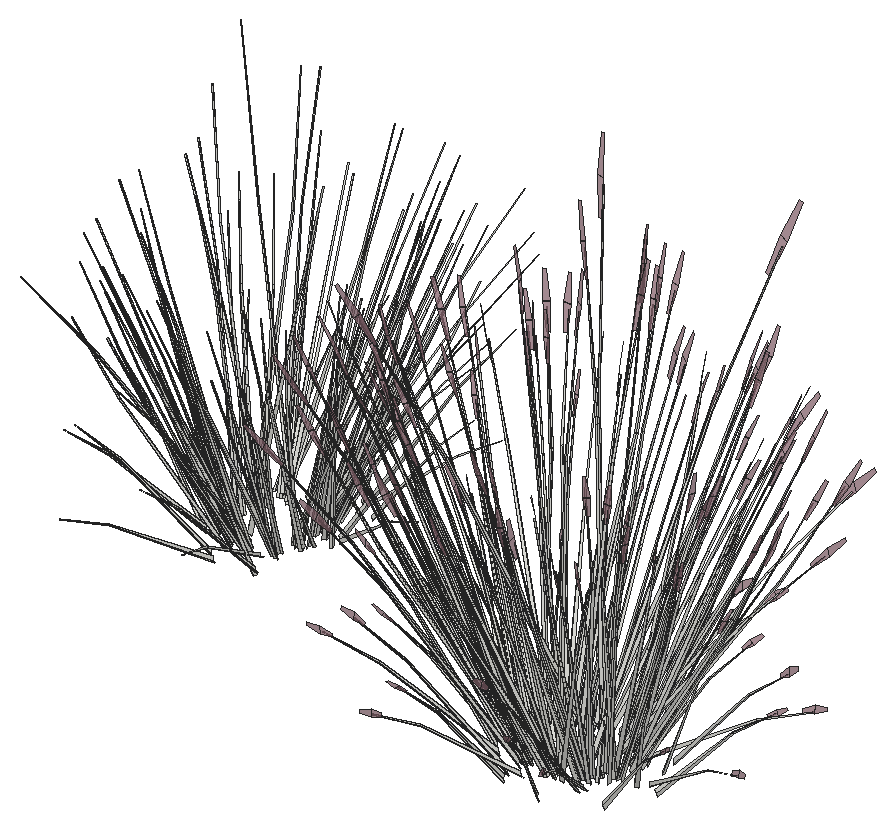
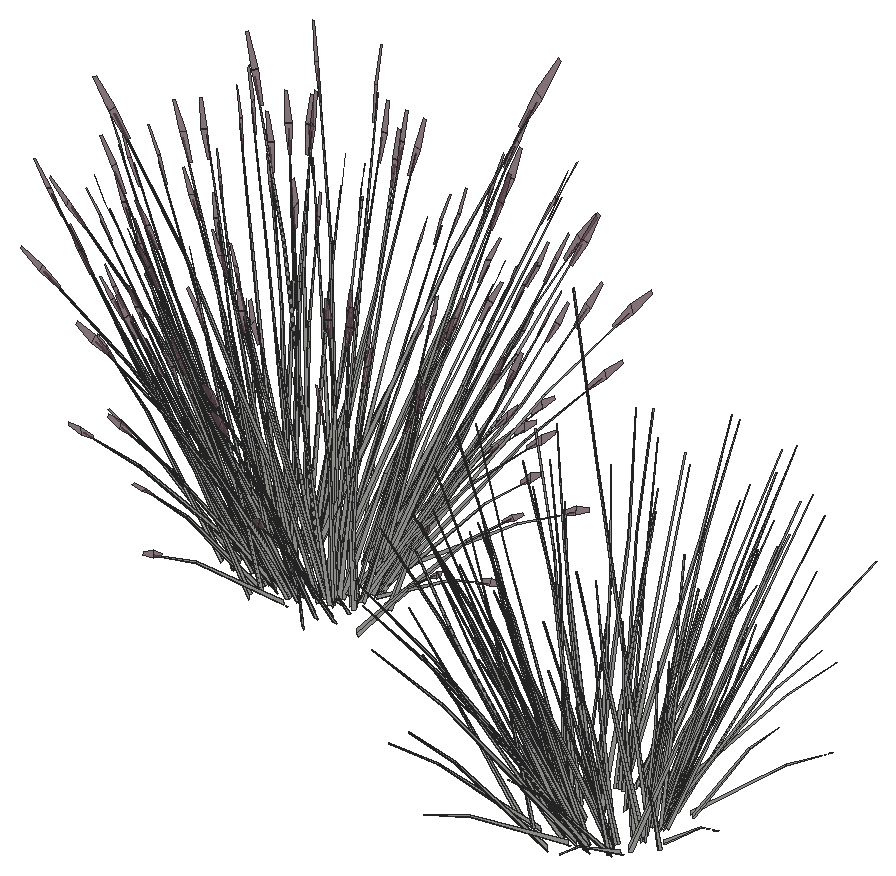
# SketchUp Ruby script. Lengths in inches.
U = 1.inch
M = Sketchup.active_model
def pt(a) = Geom::Point3d.new(a.map { |v| v * U })
def face(e, loops, mat)
  f = e.add_face(loops[0].map { |a| pt(a) })
  loops[1..].each { |l| e.add_face(l.map { |a| pt(a) }).erase! }
  f.material = f.back_material = mat if mat
  f
end
# faces: each face lists its corners as indices into pts; further lists are holes
def faces(e, pts, list, mat = nil) = list.each { |f| face(e, (f[0].is_a?(Array) ? f : [f]).map { |l| l.map { |i| pts[i] } }, mat) }
# xy, xz, yz: faces in a plane at the given z, y or x. An outline is a flat list of corners, or four numbers for a rectangle; further outlines are holes
def ring(l) = l.size == 4 ? [[l[0], l[1]], [l[2], l[1]], [l[2], l[3]], [l[0], l[3]]] : l.each_slice(2).to_a
def flat(e, list, mat, &to3) = list.each { |f| face(e, (f[0].is_a?(Array) ? f : [f]).map { |l| ring(l).map { |u, v| to3.(u, v) } }, mat) }
def xy(e, z, list, mat = nil) = flat(e, list, mat) { |x, y| [x, y, z] }
def xz(e, y, list, mat = nil) = flat(e, list, mat) { |x, z| [x, y, z] }
def yz(e, x, list, mat = nil) = flat(e, list, mat) { |y, z| [x, y, z] }
def lines(e, pts, list) = list.each { |a, b| e.add_line(pt(pts[a]), pt(pts[b])) }
# prism: a flat outline (further loops are holes) pulled along v
def prism(e, loops, v, mat = nil)
  f = face(e, loops, mat); d = Geom::Vector3d.new(v.map { |x| x * U })
  f.pushpull(f.normal.samedirection?(d) ? d.length : -d.length)
end
def box(e, o, s, mat = nil) = prism(e, [[o, [o[0] + s[0], o[1], o[2]], [o[0] + s[0], o[1] + s[1], o[2]], [o[0], o[1] + s[1], o[2]]]], [0, 0, s[2]], mat)
def at(x, y, z, deg = 0) = Geom::Transformation.translation(pt([x, y, z])) * Geom::Transformation.rotation(ORIGIN, Z_AXIS, deg.degrees)
def axes(o, x, y, z) = Geom::Transformation.new([*x, 0, *y, 0, *z, 0, *pt(o).to_a, 1])
def part(name) = M.definitions.add(name)
# library, detail: a bought-in or finely detailed component or shape, given as its bounding box
def library(name, o, s) = part(name).tap { |d| box(d.entities, o, s) }
def detail(e, o, s) = box(e.add_group.entities, o, s)
def put(e, d, t, mat = nil) = e.add_instance(d, t).tap { |i| i.material = mat if mat }
def group(e, t, mat = nil) = e.add_group.tap { |g| g.transformation = t; g.material = mat if mat }.entities
root = M.entities
M.materials.add("LightPink_Translucent").color = [144, 107, 117]
M.materials["LightPink_Translucent"].alpha = 0.75
c1 = part("blade")
p = [[2.15,0.21,22],[0,0.17,0],[0.09,0.45,0],[2.18,0.31,22],[2.29,0.31,22],[0.38,0.45,0],
  [2.48,0.24,33],[2.49,0.24,33],[2.48,0.22,33]]
faces(c1.entities,p,[[0,1,2,3],[4,5,2,3],[6,3,4,7],[8,0,3,6]])
c2 = part("blade with seeds\#1")
put(c2.entities,c1,at(0,0,0))
c3 = part("seeds")
p = [[0.3,-0.1,1.38],[-0.01,-0.03,1.59],[-0.01,-0.03,0.03],[0.14,-0.07,-0.07],[0.29,-0.03,3],[0.15,0.01,3.11]]
faces(c3.entities,p,[[0,1,2,3],[1,0,4,5]],"LightPink_Translucent")
c4 = part("blade with seeds")
put(c4.entities,c1,at(0,0,0))
put(c4.entities,c3,axes([2.4,0.25,30.99],[1.5799,-0.05474,1.17369],[-0.12525,1.92788,0.29478],[-0.07173,-0.02425,1.56792]))
put(root,c2,axes([223.65,281.09,147.9375],[0.65648,-0.82762,-0.51132],[0.57493,0.87428,-0.39606],[0.33354,0.12593,0.97836]))
put(root,c2,axes([224.63,281.77,146.46],[-0.50438,-0.0254,1.3914],[0.26641,-1.14247,0.19228],[0.53755,0.09899,0.65702]))
put(root,c2,axes([222.22,277.76,146.42],[0.39398,-0.99907,1.36359],[0.84877,0.97875,0.53923],[-0.50305,0.4384,1.14314]))
put(root,c4,axes([267.83,261.96,146.64],[0.59459,-0.93321,0.44739],[1.23546,0.44912,-0.21531],[0,0.21512,1.43643]))
put(root,c4,axes([264.97,261.54,146.64],[-1.33077,0.06393,0.44739],[-0.12035,-1.06125,-0.21531],[0.23824,-0.10756,1.43643]))
put(root,c4,axes([266.56,261.1,146.64],[-0.73619,-0.86927,0.44739],[1.11511,-0.61213,-0.21531],[0.23824,0.10756,1.43643]))
put(root,c4,axes([264.65,262.83,146.64],[-0.59459,0.93321,0.44739],[-1.23546,-0.44912,-0.21531],[0,-0.21512,1.43643]))
put(root,c4,axes([267.52,263.26,146.64],[1.33077,-0.06393,0.44739],[0.12035,1.06125,-0.21531],[-0.23824,0.10756,1.43643]))
put(root,c4,axes([269.91,266.95,146.59],[-0.78586,-0.03248,1.0506],[0.51898,-0.68985,0.58006],[0.31045,0.24509,0.8241]))
put(root,c4,axes([259.4375,260.93,146.6875],[0.78239,-0.07411,1.1486],[-0.49629,0.65296,0.84392],[-0.38663,-0.09795,0.25299]))
put(root,c4,axes([269.8,265.59,146.6875],[-0.69001,-0.29779,1.1486],[0.89096,-0.30257,0.84392],[0.24031,0.2563,0.25299]))
put(root,c4,axes([258.33,266.09,146.6875],[0.51072,-0.46938,1.1486],[0.20153,0.74307,0.84392],[-0.36908,0.13305,0.25299]))
put(root,c4,axes([274.01,263.14,146.6875],[-0.75718,0.17097,1.1486],[0.35641,-0.70661,0.84392],[0.40168,0.04835,0.25299]))
put(root,c4,axes([262.4375,256.66,146.6875],[0.63926,0.36046,1.1486],[-0.93099,0.21668,0.84392],[-0.1992,-0.27702,0.25299]))
put(root,c4,axes([262.66,268.14,146.6875],[-0.03171,-0.6158,1.1486],[0.7925,0.43922,0.84392],[-0.15586,0.29352,0.25299]))
put(root,c4,axes([272.0625,258.56,146.6875],[-0.40819,0.5272,1.1486],[-0.35086,-0.70831,0.84392],[0.33713,-0.17749,0.25299]))
put(root,c4,axes([266.92,255.9375,146.6875],[0.15721,0.60392,1.1486],[-0.87211,-0.33448,0.84392],[0.09385,-0.30923,0.25299]))
put(root,c4,axes([268.12,262.24,146.77],[-0.03348,-0.97511,1.41272],[1.51511,0.25277,0.59816],[-0.35835,0.53357,1.3335]))
put(root,c2,axes([223.15,273.86,147.51],[0.61172,-0.65782,-0.31925],[0.57907,0.75112,0.41216],[0.08811,-0.38163,0.78863]))
put(root,c2,axes([219.76,283.99,147.51],[-0.27256,0.96081,-0.31925],[-0.79518,-0.28024,0.41216],[0.07291,0.38684,0.78863]))
put(root,c2,axes([222.05,283.64,147.51],[0.13963,1.00636,-0.31925],[-0.79822,0.26574,0.41216],[0.2144,0.28839,0.78863]))
put(root,c2,axes([221.02,272.69,147.51],[0.27256,-0.96081,-0.31925],[0.79518,0.28024,0.41216],[-0.07291,-0.38684,0.78863]))
put(root,c2,axes([216.25,280.46,147.51],[-0.78697,0.17856,-0.31925],[-0.2078,-1.02074,0.41216],[-0.22552,0.27417,0.78863]))
put(root,c2,axes([223.9,281.87,147.51],[0.51441,0.78225,-0.31925],[-0.58738,0.7405,0.41216],[0.29843,0.11267,0.78863]))
put(root,c2,axes([218.73,273.05,147.51],[-0.13963,-1.00636,-0.31925],[0.79822,-0.26574,0.41216],[-0.2144,-0.28839,0.78863]))
put(root,c2,axes([224.81,279.15,147.51],[0.75135,0.34854,-0.31925],[-0.21915,1.01686,0.41216],[0.30251,-0.09324,0.78863]))
put(root,c2,axes([216.88,274.82,147.51],[-0.51441,-0.78225,-0.31925],[0.58738,-0.7405,0.41216],[-0.29843,-0.11267,0.78863]))
put(root,c2,axes([215.97,277.53,147.51],[-0.75135,-0.34854,-0.31925],[0.21915,-1.01686,0.41216],[-0.30251,0.09324,0.78863]))
put(root,c2,axes([217.63,282.83,147.51],[-0.61172,0.65782,-0.31925],[-0.57907,-0.75112,0.41216],[-0.08811,0.38163,0.78863]))
put(root,c2,axes([223.24,271.9,146.97],[-0.82131,0.22128,-0.03148],[-0.18882,-1.04586,-0.14272],[0.05207,-0.2184,0.47074]))
put(root,c4,axes([263.98,258.57,148.91],[-1.04497,-0.50058,-0.71045],[0.74264,-0.8772,0.08574],[-0.3786,-0.29889,1.00501]))
put(root,c4,axes([265.12,266.26,148.91],[0.5849,0.8421,-0.71045],[-1.20401,0.4693,0.08574],[0.13677,0.40688,1.00501]))
put(root,c4,axes([261.85,259.81,148.91],[-1.22504,-0.02494,-0.71045],[0.08228,-1.05005,0.08574],[-0.51899,-0.11081,1.00501]))
put(root,c4,axes([270.63,260.82,148.91],[0.64013,-0.81717,-0.71045],[1.12174,0.58074,0.08574],[0.38221,-0.29607,1.00501]))
put(root,c4,axes([270.9375,262.88,148.91],[1.07686,-0.45739,-0.71045],[0.60013,0.94154,0.08574],[0.52031,-0.10696,1.00501]))
put(root,c4,axes([269.05,259.16,148.91],[0.03189,-0.95798,-0.71045],[1.34277,0.06434,0.08574],[0.14171,-0.40585,1.00501]))
put(root,c4,axes([269.88,264.79,148.91],[1.22504,0.02494,-0.71045],[-0.08228,1.05005,0.08574],[0.51899,0.11081,1.00501]))
put(root,c4,axes([266.61,258.33,148.91],[-0.5849,-0.8421,-0.71045],[1.20401,-0.4693,0.08574],[-0.13677,-0.40688,1.00501]))
put(root,c2,axes([221.58,276.22,146.92],[-0.16834,0.42944,1.54493],[-0.70619,-0.88871,0.12492],[0.31858,-0.5539,0.66044]))
put(root,c2,axes([216.97,276.76,146.92],[0.33582,0.21526,1.54493],[-0.69497,0.90306,0.12492],[-0.43315,-0.40739,0.66044]))
put(root,c2,axes([220.04,275.3125,146.92],[0.02213,0.47954,1.54493],[-0.95907,-0.31812,0.12492],[0.05932,-0.68338,0.66044]))
put(root,c2,axes([222.56,277.99,146.92],[-0.31369,0.26428,1.54493],[-0.26409,-1.22118,0.12492],[0.49247,-0.276,0.66044]))
put(root,c2,axes([222.71,280.15,146.92],[-0.375,0.0283,1.54493],[0.24877,-1.22643,0.12492],[0.53441,0.07586,0.66044]))
put(root,c2,axes([222,282.11,146.92],[-0.33582,-0.21526,1.54493],[0.69497,-0.90306,0.12492],[0.43315,0.40739,0.66044]))
put(root,c2,axes([220.62,283.37,146.92],[-0.20666,-0.40114,1.54493],[0.95496,-0.33772,0.12492],[0.21583,0.62976,0.66044]))
put(root,c2,axes([221.26,281.9,146.92],[-0.3002,-0.28876,1.54493],[0.81031,-0.72911,0.12492],[0.36902,0.50009,0.66044]))
put(root,c2,axes([216.42,280.89,146.92],[0.31369,-0.26428,1.54493],[0.26409,1.22118,0.12492],[-0.49247,0.276,0.66044]))
put(root,c2,axes([217.39,282.66,146.92],[0.16834,-0.42944,1.54493],[0.70619,0.88871,0.12492],[-0.31858,0.5539,0.66044]))
put(root,c2,axes([218.93,283.57,146.92],[-0.02213,-0.47954,1.54493],[0.95907,0.31812,0.12492],[-0.05932,0.68338,0.66044]))
put(root,c4,axes([265.56,266.43,148.61],[1.20468,0.25962,-0.51099],[-0.41292,0.89013,-0.3958],[0.11046,0.35838,0.97773]))
put(root,c4,axes([268.78,258.84,148.61],[-0.87728,-0.69587,-0.51099],[0.92674,-0.60943,-0.3958],[0.13348,-0.35356,0.97773]))
put(root,c4,axes([263.49,258.6,148.61],[-1.20928,0.24619,-0.51099],[-0.21154,-0.93233,-0.3958],[-0.32481,-0.26718,0.97773]))
put(root,c4,axes([271.15,262.54,148.61],[0.332,-0.94205,-0.51099],[1.13828,0.3229,-0.3958],[0.45829,-0.08638,0.97773]))
put(root,c4,axes([261.44,260.02,148.61],[-0.88986,0.68603,-0.51099],[-0.77932,-0.72471,-0.3958],[-0.45212,-0.10438,0.97773]))
put(root,c4,axes([261.13,264.16,148.61],[0.31482,0.94565,-0.51099],[-1.19224,0.16542,-0.3958],[-0.34166,0.254,0.97773]))
put(root,c4,axes([260.58,262.06,148.61],[-0.332,0.94205,-0.51099],[-1.13828,-0.3229,-0.3958],[-0.45829,0.08638,0.97773]))
put(root,c4,axes([266.18,258.16,148.61],[-1.20468,-0.25962,-0.51099],[0.41292,-0.89013,-0.3958],[-0.11046,-0.35838,0.97773]))
put(root,c4,axes([270.6,260.44,148.61],[-0.31482,-0.94565,-0.51099],[1.19224,-0.16542,-0.3958],[0.34166,-0.254,0.97773]))
put(root,c4,axes([268.24,266,148.61],[1.20928,-0.24619,-0.51099],[0.21154,0.93233,-0.3958],[0.32481,0.26718,0.97773]))
put(root,c4,axes([262.68,265.44,149.26],[-0.03189,0.95798,-0.7886],[-1.34277,-0.06434,0.09517],[-0.14171,0.40585,1.11556]))
put(root,c4,axes([262.96,265.76,148.93],[0.87728,0.69587,-0.5672],[-0.92674,0.60943,-0.43934],[-0.13348,0.35356,1.08528]))
put(root,c4,axes([266.48,264.24,147.25],[1.05902,0.41762,1.51261],[-1.03748,0.89969,0.59816],[-0.46471,-0.53324,1.26806]))
put(root,c4,axes([262.98,261.49,147.27],[0.34834,-0.14982,1.77064],[0.12012,1.04605,0.13857],[-0.75452,0.1388,0.63284]))
put(root,c4,axes([262.23,266.79,147.29],[0.02693,-0.53464,1.54345],[1.21102,0.2824,0.21329],[-0.10493,0.5698,0.72882]))
put(root,c4,axes([270.62,265.22,148.45],[0.69728,0.64842,-0.35414],[-0.79619,0.61382,0.4572],[0.40453,0.09339,0.87481]))
put(root,c4,axes([259.88,261.63,148.45],[-1.01846,-0.28891,-0.35414],[0.29705,-0.84289,0.4572],[-0.41005,0.07729,0.87481]))
put(root,c4,axes([260.25,264.06,148.45],[-1.06674,0.14801,-0.35414],[-0.28168,-0.84611,0.4572],[-0.30569,0.22726,0.87481]))
put(root,c4,axes([271.85,262.97,148.45],[1.01846,0.28891,-0.35414],[-0.29705,0.84289,0.4572],[0.41005,-0.07729,0.87481]))
put(root,c4,axes([263.62,257.91,148.45],[-0.18927,-0.83419,-0.35414],[1.08199,-0.22027,0.4572],[-0.29062,-0.23905,0.87481]))
put(root,c4,axes([262.13,266.02,148.45],[-0.82919,0.54528,-0.35414],[-0.78493,-0.62262,0.4572],[-0.11943,0.31634,0.87481]))
put(root,c4,axes([271.48,260.54,148.45],[1.06674,-0.14801,-0.35414],[0.28168,0.84611,0.4572],[0.30569,-0.22726,0.87481]))
put(root,c4,axes([265.01,266.98,148.45],[-0.36946,0.79643,-0.35414],[-1.07787,-0.23229,0.4572],[0.09883,0.32066,0.87481]))
put(root,c4,axes([269.6,258.58,148.45],[0.82919,-0.54528,-0.35414],[0.78493,0.62262,0.4572],[0.11943,-0.31634,0.87481]))
put(root,c4,axes([266.72,257.62,148.45],[0.36946,-0.79643,-0.35414],[1.07787,0.23229,0.4572],[-0.09883,-0.32066,0.87481]))
put(root,c4,axes([261.11,259.38,148.45],[-0.69728,-0.64842,-0.35414],[0.79619,-0.61382,0.4572],[-0.40453,-0.09339,0.87481]))
put(root,c2,axes([223.22,274.61,147.97],[-0.99362,-0.0619,-0.10962],[0.02716,-1.17208,-0.60845],[0.06902,-0.45141,0.92453]))
put(root,c2,axes([219.4,283.38,147.97],[0.88471,-0.5817,-0.10962],[0.43476,1.03242,-0.60845],[0.11673,0.43507,0.92453]))
put(root,c2,axes([217.47,274.73,147.97],[-0.04841,1.27062,-0.10962],[-0.91657,-0.03473,-0.60845],[-0.353,-0.08826,0.92453]))
put(root,c2,axes([221.38,273.3,147.97],[-0.88471,0.5817,-0.10962],[-0.43476,-1.03242,-0.60845],[-0.11673,-0.43507,0.92453]))
put(root,c2,axes([224.33,279.6,147.97],[-0.45489,-1.13134,-0.10962],[0.80735,-0.55596,-0.60845],[0.34022,-0.14927,0.92453]))
put(root,c2,axes([217.56,282.07,147.97],[0.99362,0.0619,-0.10962],[-0.02716,1.17208,-0.60845],[-0.06902,0.45141,0.92453]))
put(root,c2,axes([224.3,276.92,147.97],[-0.8363,-0.68892,-0.10962],[0.4818,-0.99769,-0.60845],[0.23628,-0.3468,0.92453]))
put(root,c2,axes([221.51,283.34,147.97],[0.53874,-1.06944,-0.10962],[0.78019,0.61612,-0.60845],[0.2712,0.30214,0.92453]))
put(root,c2,axes([216.45,277.08,147.97],[0.45489,1.13134,-0.10962],[-0.80735,0.55596,-0.60845],[-0.34022,0.14927,0.92453]))
put(root,c2,axes([219.28,273.34,147.97],[-0.53874,1.06944,-0.10962],[-0.78019,-0.61612,-0.60845],[-0.2712,-0.30214,0.92453]))
put(root,c2,axes([219.36,276.14,147.46],[-0.50765,0.99901,1.24659],[-0.79039,-1.05487,0.53787],[0.47632,-0.32232,1.20495]))
put(root,c2,axes([220.29,284.59,147.68],[0.12685,0.18879,1.57709],[0.92682,-0.01606,-0.24942],[0.12053,0.43275,0.12648]))
put(root,c2,axes([219.99,270.14,147.68],[-0.14882,-0.16043,1.57709],[-0.91289,0.20534,-0.24942],[-0.17308,-0.40254,0.12648]))
put(root,c2,axes([222.62,273.59,147.68],[-0.01652,-0.24801,1.57709],[-0.75906,-0.68026,-0.24942],[0.1002,-0.44114,0.12648]))
put(root,c2,axes([216.02,273.57,147.68],[-0.19445,0.01116,1.57709],[-0.562,0.94258,-0.24942],[-0.34067,-0.14573,0.12648]))
put(root,c2,axes([223.75,284.5625,147.68],[0.19335,0.02874,1.57709],[0.67262,-0.81555,-0.24942],[0.31807,0.21351,0.12648]))
put(root,c2,axes([226.14,279.87,147.68],[0.15733,-0.14655,1.57709],[0.06181,-1.18266,-0.24942],[0.34698,-0.11893,0.12648]))
put(root,c2,axes([214.34,278.875,147.68],[-0.13699,0.17683,1.57709],[0.08685,1.18009,-0.24942],[-0.32765,0.18834,0.12648]))
put(root,c2,axes([215.84,282.74,147.68],[-0.0069,0.24875,1.57709],[0.68965,0.79195,-0.24942],[-0.14092,0.42256,0.12648]))
put(root,c2,axes([216.43,283.7,147.67],[0.0975,-0.08571,1.59908],[0.87648,0.41319,-0.1511],[0.00634,0.41846,0.28298]))
put(root,c2,axes([213.89,280.08,147.67],[0.11711,0.02157,1.59908],[0.42502,1.06376,-0.1511],[-0.21726,0.31303,0.28298]))
put(root,c2,axes([224.99,277.82,147.67],[-0.11829,-0.00342,1.59908],[-0.52187,-0.99076,-0.1511],[0.18628,-0.34414,0.28298]))
put(root,c2,axes([221.22,286.69,147.67],[0.0262,-0.14755,1.59908],[0.86326,-0.45644,-0.1511],[0.22658,0.30203,0.28298]))
put(root,c2,axes([219.04,270.71,147.67],[-0.00742,0.151,1.59908],[-0.79509,0.62706,-0.1511],[-0.26143,-0.25182,0.28298]))
put(root,c2,axes([224.01,270.99,147.67],[-0.08553,0.10454,1.59908],[-0.91687,-0.22868,-0.1511],[-0.05858,-0.41178,0.28298]))
put(root,c2,axes([225.73,284.65,147.67],[-0.05899,-0.13116,1.59908],[0.39237,-1.08407,-0.1511],[0.32669,0.02548,0.28298]))
put(root,c2,axes([215.32,273.82,147.67],[0.07463,0.11741,1.59908],[-0.25178,1.15035,-0.1511],[-0.32567,0.04164,0.28298]))
put(root,c4,axes([272.7,265.32,147.85],[-0.23455,-0.87059,-0.03492],[1.10861,-0.20015,-0.15832],[0.23151,0.05519,0.52218]))
put(root,c2,axes([223.31,281.95,148.29],[0.04841,-1.27062,-0.12168],[0.91657,0.03473,-0.67538],[0.353,0.08826,1.02623]))
put(root,c2,axes([216.11,279.78,148.32],[0.93666,0.77159,-0.12278],[-0.53962,1.11741,-0.68147],[-0.26463,0.38842,1.03548]))
put(root,c2,axes([216.15,277.41,147.69],[0.25543,-1.1392,0.43274],[0.83975,0.38955,0.35681],[-0.33023,0.06846,0.89544]))
put(root,c2,axes([223.14,274.11,147.69],[0.64379,0.85247,0.43274],[-0.68369,0.73521,0.35681],[0.11875,-0.39995,0.89544]))
put(root,c2,axes([221.12,272.92,147.69],[0.89085,0.32663,0.43274],[-0.30463,1.07385,0.35681],[-0.05354,-0.4223,0.89544]))
put(root,c2,axes([221.88,283.51,147.69],[-0.89921,0.28673,0.43274],[-0.15606,-1.12475,0.35681],[0.21148,0.33149,0.89544]))
put(root,c2,axes([223.7,281.86,147.69],[-0.66663,0.82326,0.43274],[-0.57493,-0.87428,0.35681],[0.31276,0.15186,0.89544]))
put(root,c2,axes([217.08,274.82,147.69],[0.66663,-0.82326,0.43274],[0.57493,0.87428,0.35681],[-0.31276,-0.15186,0.89544]))
put(root,c2,axes([219.66,283.76,147.69],[-0.89085,-0.32663,0.43274],[0.30463,-1.07385,0.35681],[0.05354,0.4223,0.89544]))
put(root,c2,axes([218.9,273.18,147.69],[0.89921,-0.28673,0.43274],[0.15606,1.12475,0.35681],[-0.21148,-0.33149,0.89544]))
put(root,c2,axes([224.43,276.4375,147.69],[0.22422,1.14989,0.43274],[-0.87956,0.19957,0.35681],[0.25922,-0.27044,0.89544]))
put(root,c2,axes([216.18,280.02,147.69],[-0.62066,-0.52545,0.05797],[0.36135,-0.74826,0.45634],[-0.19899,0.24191,0.69585]))
put(root,c2,axes([224.7,279.58,147.69],[0.33205,0.8519,0.05797],[-0.60551,0.41697,0.45634],[0.26692,-0.08227,0.69585]))
put(root,c2,axes([219.08,272.95,147.69],[0.4109,-0.79368,0.05797],[0.58514,0.46209,0.45634],[-0.18917,-0.25446,0.69585]))
put(root,c2,axes([221.36,272.84,147.69],[0.66618,-0.42462,0.05797],[0.32607,0.77431,0.45634],[-0.06434,-0.34133,0.69585]))
put(root,c2,axes([217.4,282.49,147.69],[-0.74296,-0.05822,0.05797],[0.02037,-0.87906,0.45634],[-0.07774,0.33673,0.69585]))
put(root,c2,axes([217.15,274.52,147.69],[0.04552,-0.95007,0.05797],[0.68742,0.02605,0.45634],[-0.26332,-0.09941,0.69585]))
put(root,c2,axes([223.38,274.19,147.69],[0.74296,0.05822,0.05797],[-0.02037,0.87906,0.45634],[0.07774,-0.33673,0.69585]))
put(root,c2,axes([221.7,283.73,147.69],[-0.4109,0.79368,0.05797],[-0.58514,-0.46209,0.45634],[0.18917,0.25446,0.69585]))
put(root,c2,axes([216.09,277.1,147.69],[-0.33205,-0.8519,0.05797],[0.60551,-0.41697,0.45634],[-0.26692,0.08227,0.69585]))
put(root,c2,axes([219.42,283.85,147.69],[-0.66618,0.42462,0.05797],[-0.32607,-0.77431,0.45634],[0.06434,0.34133,0.69585]))
put(root,c2,axes([224.6,276.66,147.69],[0.62066,0.52545,0.05797],[-0.36135,0.74826,0.45634],[0.19899,-0.24191,0.69585]))
put(root,c2,axes([223.63,282.17,147.69],[-0.04552,0.95007,0.05797],[-0.68742,-0.02605,0.45634],[0.26332,0.09941,0.69585]))
put(root,c2,axes([224.01,279.26,147.98],[-0.75135,-0.34854,0.31925],[0.21915,-1.01686,-0.41216],[0.30251,-0.09324,0.78863]))
put(root,c2,axes([216.77,277.42,147.98],[0.75135,0.34854,0.31925],[-0.21915,1.01686,-0.41216],[-0.30251,0.09324,0.78863]))
put(root,c2,axes([222.83,274.79,147.98],[-0.61172,0.65782,0.31925],[-0.57907,-0.75112,-0.41216],[0.08811,-0.38163,0.78863]))
put(root,c2,axes([221.11,273.71,147.98],[-0.27256,0.96081,0.31925],[-0.79518,-0.28024,-0.41216],[-0.07291,-0.38684,0.78863]))
put(root,c2,axes([217.95,281.89,147.98],[0.61172,-0.65782,0.31925],[0.57907,0.75112,-0.41216],[-0.08811,0.38163,0.78863]))
put(root,c2,axes([223.17,281.46,147.98],[-0.51441,-0.78225,0.31925],[0.58738,-0.7405,-0.41216],[0.29843,0.11267,0.78863]))
put(root,c2,axes([221.58,282.82,147.98],[-0.13963,-1.00636,0.31925],[0.79822,-0.26574,-0.41216],[0.2144,0.28839,0.78863]))
put(root,c2,axes([223.89,276.82,147.98],[-0.78697,0.17856,0.31925],[-0.2078,-1.02074,-0.41216],[0.22552,-0.27417,0.78863]))
put(root,c2,axes([219.2,273.87,147.98],[0.13963,1.00636,0.31925],[-0.79822,0.26574,-0.41216],[-0.2144,-0.28839,0.78863]))
put(root,c2,axes([219.67,282.98,147.98],[0.27256,-0.96081,0.31925],[0.79518,0.28024,-0.41216],[0.07291,0.38684,0.78863]))
put(root,c2,axes([217.61,275.23,147.98],[0.51441,0.78225,0.31925],[-0.58738,0.7405,-0.41216],[-0.29843,-0.11267,0.78863]))
put(root,c2,axes([216.89,279.86,147.98],[0.78697,-0.17856,0.31925],[0.2078,1.02074,-0.41216],[-0.22552,0.27417,0.78863]))
put(root,c4,axes([268.12,263.56,147.8],[-0.45521,-0.17844,1.71376],[0.94204,-0.74856,0.13857],[0.58713,0.33769,0.73262]))
put(root,c4,axes([267.54,258.67,147.8],[-0.22818,0.35597,1.71376],[-0.95725,-0.73667,0.13857],[0.43183,-0.45914,0.73262]))
put(root,c4,axes([269.08,261.93,147.8],[-0.50831,0.02346,1.71376],[0.33721,-1.01661,0.13857],[0.72439,0.06288,0.73262]))
put(root,c4,axes([266.24,264.6,147.8],[-0.28013,-0.33252,1.71376],[1.29445,-0.27994,0.13857],[0.29256,0.52202,0.73262]))
put(root,c4,axes([263.95,264.76,147.8],[-0.02999,-0.3975,1.71376],[1.30002,0.26369,0.13857],[-0.08041,0.56647,0.73262]))
put(root,c4,axes([261.87,264.01,147.8],[0.22818,-0.35597,1.71376],[0.95725,0.73667,0.13857],[-0.43183,0.45914,0.73262]))
put(root,c4,axes([260.54,262.54,147.8],[0.42521,-0.21906,1.71376],[0.35798,1.01226,0.13857],[-0.66754,0.22878,0.73262]))
put(root,c4,axes([262.1,263.23,147.8],[0.30609,-0.31822,1.71376],[0.77286,0.85893,0.13857],[-0.53009,0.39116,0.73262]))
put(root,c4,axes([263.16,258.09,147.8],[0.28013,0.33252,1.71376],[-1.29445,0.27994,0.13857],[-0.29256,-0.52202,0.73262]))
put(root,c4,axes([261.29,259.125,147.8],[0.45521,0.17844,1.71376],[-0.94204,0.74856,0.13857],[-0.58713,-0.33769,0.73262]))
put(root,c4,axes([260.33,260.75,147.8],[0.50831,-0.02346,1.71376],[-0.33721,1.01661,0.13857],[-0.72439,-0.06288,0.73262]))
put(root,c2,axes([224.63,279.28,147.99],[-0.25543,1.1392,0.48034],[-0.83975,-0.38955,0.39606],[0.33023,-0.06846,0.99394]))
put(root,c2,axes([217.4,282.92,148.02],[-0.72104,-0.95477,0.48466],[0.76573,-0.82343,0.39963],[-0.133,0.44794,1.00289]))
put(root,c2,axes([215.97,280.32,148.02],[-0.25113,-1.28788,0.48466],[0.9851,-0.22351,0.39963],[-0.29033,0.30289,1.00289]))
put(root,c2,axes([226.69,277.89,148.52],[-0.56051,-0.79893,-0.05849],[0.61388,-0.73204,-0.26518],[0.17394,-0.05154,0.87466]))
put(root,c2,axes([223.84,285.1,148.52],[0.2608,-1.0202,-0.05849],[0.8027,0.31383,-0.26518],[0.12187,0.16686,0.87466]))
put(root,c4,axes([269.82,265.29,148.96],[0.06562,-1.05324,-0.1216],[1.2424,0.02879,-0.67495],[0.4785,0.07316,1.02557]))
put(root,c4,axes([260.52,261.25,148.96],[0.6166,0.93779,-0.1216],[-1.09436,0.46085,-0.67495],[-0.46117,0.12373,1.02557]))
put(root,c4,axes([269.7,259.21,148.96],[-1.34686,-0.05131,-0.1216],[0.03681,-0.97156,-0.67495],[0.09356,-0.37418,1.02557]))
put(root,c4,axes([271.21,263.35,148.96],[-0.6166,-0.93779,-0.1216],[1.09436,-0.46085,-0.67495],[0.46117,-0.12373,1.02557]))
put(root,c4,axes([264.53,266.48,148.96],[1.19922,-0.48218,-0.1216],[0.58932,0.85579,-0.67495],[0.15822,0.36063,1.02557]))
put(root,c4,axes([261.91,259.3,148.96],[-0.06562,1.05324,-0.1216],[-1.2424,-0.02879,-0.67495],[-0.4785,-0.07316,1.02557]))
put(root,c4,axes([267.38,266.44,148.96],[0.73026,-0.88648,-0.1216],[1.05755,0.51071,-0.67495],[0.36761,0.25045,1.02557]))
put(root,c4,axes([260.57,263.48,148.96],[1.1336,0.57106,-0.1216],[-0.65308,0.827,-0.67495],[-0.32027,0.28747,1.02557]))
put(root,c4,axes([267.21,258.12,148.96],[-1.19922,0.48218,-0.1216],[-0.58932,-0.85579,-0.67495],[-0.15822,-0.36063,1.02557]))
put(root,c4,axes([271.16,261.12,148.96],[-1.1336,-0.57106,-0.1216],[0.65308,-0.827,-0.67495],[0.32027,-0.28747,1.02557]))
put(root,c4,axes([268.2,261.21,148.4],[-1.05895,-0.53811,1.38283],[1.11816,-0.83781,0.59665],[0.34166,0.5049,1.33663]))
put(root,c4,axes([259.24,262.1875,148.64],[-0.20012,0.13446,1.74944],[0.01702,0.98243,-0.27667],[-0.45871,0.12776,0.14031]))
put(root,c4,axes([274.56,261.875,148.64],[0.17006,-0.15775,1.74944],[-0.21766,-0.96766,-0.27667],[0.42669,-0.18347,0.14031]))
put(root,c4,axes([270.9,264.66,148.64],[0.26289,-0.01751,1.74944],[0.72108,-0.8046,-0.27667],[0.46761,0.10621,0.14031]))
put(root,c4,axes([270.92,257.66,148.64],[-0.01183,-0.20612,1.74944],[-0.99913,-0.59572,-0.27667],[0.15447,-0.36112,0.14031]))
put(root,c4,axes([259.27,265.86,148.64],[-0.03046,0.20495,1.74944],[0.86449,0.71297,-0.27667],[-0.22632,0.33716,0.14031]))
put(root,c4,axes([264.24,268.39,148.64],[0.15534,0.16677,1.74944],[1.25362,0.06552,-0.27667],[0.12606,0.3678,0.14031]))
put(root,c4,axes([265.3,255.88,148.64],[-0.18744,-0.14521,1.74944],[-1.25089,0.09206,-0.27667],[-0.19964,-0.34731,0.14031]))
put(root,c4,axes([261.2,257.48,148.64],[-0.26368,-0.00731,1.74944],[-0.83946,0.73103,-0.27667],[-0.44791,-0.14937,0.14031]))
put(root,c4,axes([260.1875,258.1,148.63],[0.09085,0.10335,1.77383],[-0.43798,0.92907,-0.16761],[-0.44357,0.00672,0.31391]))
put(root,c4,axes([264.02,255.41,148.63],[-0.02286,0.12414,1.77383],[-1.12758,0.45052,-0.16761],[-0.33182,-0.23029,0.31391]))
put(root,c4,axes([266.42,267.18,148.63],[0.00363,-0.12539,1.77383],[1.0502,-0.55319,-0.16761],[0.36479,0.19745,0.31391]))
put(root,c4,axes([257.01,263.18,148.63],[0.1564,0.02778,1.77383],[0.48382,0.91506,-0.16761],[-0.32016,0.24017,0.31391]))
put(root,c4,axes([273.95,260.87,148.63],[-0.16006,-0.00787,1.77383],[-0.66468,-0.8428,-0.16761],[0.26693,-0.27711,0.31391]))
put(root,c4,axes([273.66,266.13,148.63],[-0.11081,-0.09067,1.77383],[0.2424,-0.97188,-0.16761],[0.43649,-0.06209,0.31391]))
put(root,c4,axes([259.17,267.96,148.63],[0.13903,-0.06253,1.77383],[1.14912,0.41591,-0.16761],[-0.027,0.34629,0.31391]))
put(root,c4,axes([270.65,256.92,148.63],[-0.12446,0.07911,1.77383],[-1.21937,-0.26689,-0.16761],[-0.04414,-0.34521,0.31391]))
put(root,c4,axes([262.04,265.39,149.32],[1.34686,0.05131,-0.13498],[-0.03681,0.97156,-0.74919],[-0.09356,0.37418,1.13838]))
put(root,c4,axes([264.34,257.77,149.35],[-0.81789,0.99285,-0.13619],[-1.18445,-0.572,-0.75594],[-0.41173,-0.28051,1.14864]))
put(root,c4,axes([264.09,257.83,148.65],[0.55698,-0.6579,0.0643],[0.79316,0.38303,0.50621],[-0.25643,-0.21093,0.77189]))
put(root,c4,axes([264.55,266.86,148.65],[-0.90301,0.35198,0.0643],[-0.44199,-0.64184,0.50621],[0.08721,0.28293,0.77189]))
put(root,c4,axes([271.58,260.91,148.65],[0.8413,0.43556,0.0643],[-0.48981,0.62025,0.50621],[0.26973,-0.20053,0.77189]))
put(root,c4,axes([271.7,263.33,148.65],[0.4501,0.70615,0.0643],[-0.82077,0.34564,0.50621],[0.36181,-0.0682,0.77189]))
put(root,c4,axes([261.47,259.13,148.65],[0.06171,-0.78753,0.0643],[0.9318,0.02159,0.50621],[-0.35694,-0.08241,0.77189]))
put(root,c4,axes([269.92,258.86,148.65],[1.00708,0.04826,0.0643],[-0.02761,0.72867,0.50621],[0.10538,-0.27912,0.77189]))
put(root,c4,axes([270.26,265.47,148.65],[-0.06171,0.78753,0.0643],[-0.9318,-0.02159,0.50621],[0.35694,0.08241,0.77189]))
put(root,c4,axes([260.16,263.69,148.65],[-0.8413,-0.43556,0.0643],[0.48981,-0.62025,0.50621],[-0.26973,0.20053,0.77189]))
put(root,c4,axes([267.18,257.74,148.65],[0.90301,-0.35198,0.0643],[0.44199,0.64184,0.50621],[-0.08721,-0.28293,0.77189]))
put(root,c4,axes([260.03,261.27,148.65],[-0.4501,-0.70615,0.0643],[0.82077,-0.34564,0.50621],[-0.36181,0.0682,0.77189]))
put(root,c4,axes([267.65,266.76,148.65],[-0.55698,0.6579,0.0643],[-0.79316,-0.38303,0.50621],[0.25643,0.21093,0.77189]))
put(root,c4,axes([261.8125,265.74,148.65],[-1.00708,-0.04826,0.0643],[0.02761,-0.72867,0.50621],[-0.10538,0.27912,0.77189]))
put(root,c4,axes([266.86,257.8,148.66],[1.20755,0.27075,0.48003],[-0.41292,0.89013,0.3958],[-0.07257,-0.35005,0.9933]))
put(root,c4,axes([270.35,265.22,148.66],[-0.90362,0.68241,0.48003],[-0.77932,-0.72471,0.3958],[0.42395,0.12588,0.9933]))
put(root,c4,axes([271.62,263.07,148.66],[-0.34623,0.9443,0.48003],[-1.13828,-0.3229,0.3958],[0.44763,-0.05675,0.9933]))
put(root,c4,axes([260.39,263.875,148.66],[-0.30393,-0.95317,0.48003],[1.19224,-0.16542,0.3958],[-0.35138,0.22417,0.9933]))
put(root,c4,axes([262.13,265.8,148.66],[-0.87265,-0.70663,0.48003],[0.92674,-0.60943,0.3958],[-0.16097,0.33153,0.9933]))
put(root,c4,axes([269.6,258.79,148.66],[0.87265,0.70663,0.48003],[-0.92674,0.60943,0.3958],[0.16097,-0.33153,0.9933]))
put(root,c4,axes([260.12,261.52,148.66],[0.34623,-0.9443,0.48003],[1.13828,0.3229,0.3958],[-0.44763,0.05675,0.9933]))
put(root,c4,axes([271.34,260.72,148.66],[0.30393,0.95317,0.48003],[-1.19224,0.16542,0.3958],[0.35138,-0.22417,0.9933]))
put(root,c4,axes([267.88,266.58,148.66],[-1.21888,0.23767,0.48003],[-0.21154,-0.93233,0.3958],[0.28666,0.27478,0.9933]))
put(root,c4,axes([264.89,266.14,148.98],[0.36946,-0.79643,0.35414],[1.07787,0.23229,-0.4572],[0.09883,0.32066,0.87481]))
put(root,c4,axes([266.84,258.46,148.98],[-0.36946,0.79643,0.35414],[-1.07787,-0.23229,-0.4572],[-0.09883,-0.32066,0.87481]))
put(root,c4,axes([269.63,264.88,148.98],[-0.69728,-0.64842,0.35414],[0.79619,-0.61382,-0.4572],[0.40453,0.09339,0.87481]))
put(root,c4,axes([270.78,263.0625,148.98],[-1.01846,-0.28891,0.35414],[0.29705,-0.84289,-0.4572],[0.41005,-0.07729,0.87481]))
put(root,c4,axes([262.1,259.72,148.98],[0.69728,0.64842,0.35414],[-0.79619,0.61382,-0.4572],[-0.40453,-0.09339,0.87481]))
put(root,c4,axes([262.5625,265.24,148.98],[0.82919,-0.54528,0.35414],[0.78493,0.62262,-0.4572],[-0.11943,0.31634,0.87481]))
put(root,c4,axes([261.125,263.56,148.98],[1.06674,-0.14801,0.35414],[0.28168,0.84611,-0.4572],[-0.30569,0.22726,0.87481]))
put(root,c4,axes([267.48,266.01,148.98],[-0.18927,-0.83419,0.35414],[1.08199,-0.22027,-0.4572],[0.29062,0.23905,0.87481]))
put(root,c4,axes([270.61,261.04,148.98],[-1.06674,0.14801,0.35414],[-0.28168,-0.84611,-0.4572],[0.30569,-0.22726,0.87481]))
put(root,c4,axes([260.95,261.54,148.98],[1.01846,0.28891,0.35414],[-0.29705,0.84289,-0.4572],[-0.41005,0.07729,0.87481]))
put(root,c4,axes([269.17,259.35,148.98],[-0.82919,0.54528,0.35414],[-0.78493,-0.62262,-0.4572],[0.11943,-0.31634,0.87481]))
put(root,c4,axes([264.26,258.59,148.98],[0.18927,0.83419,0.35414],[-1.08199,0.22027,-0.4572],[-0.29062,-0.23905,0.87481]))
put(root,c4,axes([264.875,266.8,148.99],[-1.20755,-0.27075,0.53283],[0.41292,-0.89013,0.43934],[0.07257,0.35005,1.10256]))
put(root,c4,axes([261.01,259.13,149.02],[1.01205,-0.7643,0.53763],[0.87284,0.81167,0.4433],[-0.47482,-0.14098,1.11249]))
put(root,c4,axes([263.77,257.61,149.02],[1.36515,-0.26619,0.53763],[0.23692,1.04421,0.4433],[-0.32106,-0.30775,1.11249]))
put(root,c4,axes([266.34,268.98,149.57],[0.84686,-0.59414,-0.06488],[0.77596,0.65071,-0.29416],[0.05463,0.18438,0.97024]))
put(root,c4,axes([258.7,265.96,149.57],[1.08141,0.27645,-0.06488],[-0.33265,0.85086,-0.29416],[-0.17688,0.12919,0.97024]))
